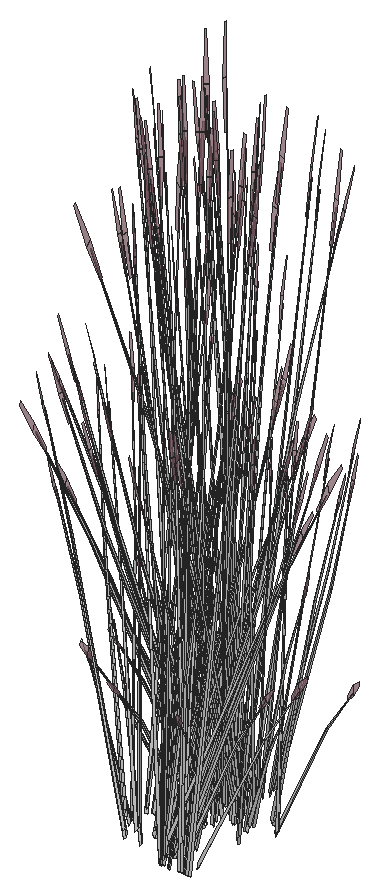
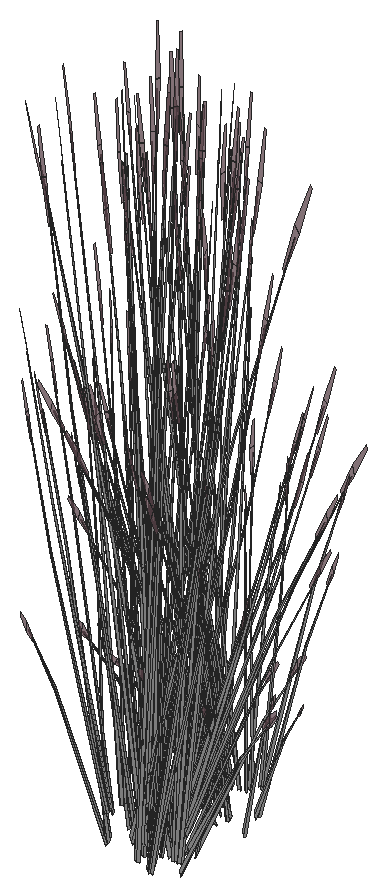
# SketchUp Ruby script. Lengths in inches.
U = 1.inch
M = Sketchup.active_model
def pt(a) = Geom::Point3d.new(a.map { |v| v * U })
def face(e, loops, mat)
  f = e.add_face(loops[0].map { |a| pt(a) })
  loops[1..].each { |l| e.add_face(l.map { |a| pt(a) }).erase! }
  f.material = f.back_material = mat if mat
  f
end
# faces: each face lists its corners as indices into pts; further lists are holes
def faces(e, pts, list, mat = nil) = list.each { |f| face(e, (f[0].is_a?(Array) ? f : [f]).map { |l| l.map { |i| pts[i] } }, mat) }
# xy, xz, yz: faces in a plane at the given z, y or x. An outline is a flat list of corners, or four numbers for a rectangle; further outlines are holes
def ring(l) = l.size == 4 ? [[l[0], l[1]], [l[2], l[1]], [l[2], l[3]], [l[0], l[3]]] : l.each_slice(2).to_a
def flat(e, list, mat, &to3) = list.each { |f| face(e, (f[0].is_a?(Array) ? f : [f]).map { |l| ring(l).map { |u, v| to3.(u, v) } }, mat) }
def xy(e, z, list, mat = nil) = flat(e, list, mat) { |x, y| [x, y, z] }
def xz(e, y, list, mat = nil) = flat(e, list, mat) { |x, z| [x, y, z] }
def yz(e, x, list, mat = nil) = flat(e, list, mat) { |y, z| [x, y, z] }
def lines(e, pts, list) = list.each { |a, b| e.add_line(pt(pts[a]), pt(pts[b])) }
# prism: a flat outline (further loops are holes) pulled along v
def prism(e, loops, v, mat = nil)
  f = face(e, loops, mat); d = Geom::Vector3d.new(v.map { |x| x * U })
  f.pushpull(f.normal.samedirection?(d) ? d.length : -d.length)
end
def box(e, o, s, mat = nil) = prism(e, [[o, [o[0] + s[0], o[1], o[2]], [o[0] + s[0], o[1] + s[1], o[2]], [o[0], o[1] + s[1], o[2]]]], [0, 0, s[2]], mat)
def at(x, y, z, deg = 0) = Geom::Transformation.translation(pt([x, y, z])) * Geom::Transformation.rotation(ORIGIN, Z_AXIS, deg.degrees)
def axes(o, x, y, z) = Geom::Transformation.new([*x, 0, *y, 0, *z, 0, *pt(o).to_a, 1])
def part(name) = M.definitions.add(name)
# library, detail: a bought-in or finely detailed component or shape, given as its bounding box
def library(name, o, s) = part(name).tap { |d| box(d.entities, o, s) }
def detail(e, o, s) = box(e.add_group.entities, o, s)
def put(e, d, t, mat = nil) = e.add_instance(d, t).tap { |i| i.material = mat if mat }
def group(e, t, mat = nil) = e.add_group.tap { |g| g.transformation = t; g.material = mat if mat }.entities
root = M.entities
M.materials.add("LightPink_Translucent").color = [144, 107, 117]
M.materials["LightPink_Translucent"].alpha = 0.75
M.materials.add("[_0053_Ivory_]").color = [200, 200, 200]
c1 = part("blade")
p = [[2.15,0.21,22],[0,0.17,0],[0.09,0.45,0],[2.18,0.31,22],[2.29,0.31,22],[0.38,0.45,0],
  [2.48,0.24,33],[2.49,0.24,33],[2.48,0.22,33]]
faces(c1.entities,p,[[0,1,2,3],[4,5,2,3],[6,3,4,7],[8,0,3,6]])
c2 = part("seeds")
p = [[0.3,-0.1,1.38],[-0.01,-0.03,1.59],[-0.01,-0.03,0.03],[0.14,-0.07,-0.07],[0.29,-0.03,3],[0.15,0.01,3.11]]
faces(c2.entities,p,[[0,1,2,3],[1,0,4,5]],"LightPink_Translucent")
c3 = part("blade with seeds")
put(c3.entities,c1,at(0,0,0))
put(c3.entities,c2,axes([2.4,0.25,30.99],[1.5799,-0.05474,1.17369],[-0.12525,1.92788,0.29478],[-0.07173,-0.02425,1.56792]))
put(root,c3,axes([629.1875,284.57,255.53],[0.21074,-0.13302,1.71376],[0.17741,0.61464,0.13857],[-0.33083,0.13891,0.73262]),"[_0053_Ivory_]")
put(root,c3,axes([633.4,292.35,256.63],[0.0158,-0.58168,-0.71045],[0.66548,0.03907,0.08574],[0.07023,-0.24643,1.00501]),"[_0053_Ivory_]")
put(root,c3,axes([632.25,291.42,256.18],[0.1831,-0.48359,-0.35414],[0.53419,0.14105,0.4572],[-0.04898,-0.1947,0.87481]),"[_0053_Ivory_]")
put(root,c3,axes([632.65,292.06,255.53],[-0.11309,0.21615,1.71376],[-0.47441,-0.44731,0.13857],[0.21402,-0.27879,0.73262]),"[_0053_Ivory_]")
put(root,c3,axes([633.82,285.9375,256.63],[0.60713,0.01514,-0.71045],[-0.04078,0.63759,0.08574],[0.25721,0.06729,1.00501]),"[_0053_Ivory_]")
put(root,c3,axes([633.13,286.45,254.13],[0.56842,-0.31443,0.49651],[0.33976,0.56381,0],[-0.12946,0.07161,1.57504]),"[_0053_Ivory_]")
put(root,c3,axes([631.98,291.75,256.33],[-0.59704,-0.15764,-0.51099],[0.20464,-0.54049,-0.3958],[-0.05475,-0.21761,0.97773]),"[_0053_Ivory_]")
put(root,c3,axes([632.35,290.4,254.42],[0.07791,0.3667,1.1486],[-0.43222,-0.2031,0.84392],[0.04651,-0.18776,0.25299]),"[_0053_Ivory_]")
put(root,c3,axes([632.32,285.95,253.94],[0.26406,0.72244,-0.06012],[-0.7545,0.25315,0],[0.00922,0.02523,1.72173]),"[_0053_Ivory_]")
put(root,c3,axes([632.62,286.73,253.68],[-0.56663,-0.1556,-0.30978],[0.14267,-0.54795,0.30978],[-0.11423,0.06319,1.38974]),"[_0053_Ivory_]")
put(root,c3,axes([633.27,292.16,256.33],[-0.43478,-0.42253,-0.51099],[0.45929,-0.37004,-0.3958],[0.06615,-0.21468,0.97773]),"[_0053_Ivory_]")
put(root,c3,axes([628.53,285.62,254.24],[0.21107,0.05162,1.43002],[0.13604,0.52729,-0.30754],[-0.28671,0.0987,0.61141]),"[_0053_Ivory_]")
put(root,c3,axes([634.81,284.64,254.03],[0.75945,0,0],[0,0.70283,-0.51607],[0,0.16007,1.63711]),"[_0053_Ivory_]")
put(root,c3,axes([634.51,285,253.85],[-0.75908,-0.00503,-0.04976],[0,-0.70283,0.49943],[-0.02386,0.16,1.58352]),"[_0053_Ivory_]")
put(root,c3,axes([632.86,284.39,254.32],[0.68399,0.30005,-0.29095],[-0.32934,0.63331,-0.50002],[0.0215,0.15549,1.59708]),"[_0053_Ivory_]")
put(root,c3,axes([628.09,286.73,254.42],[0.25312,-0.28501,1.1486],[0.09988,0.45119,0.84392],[-0.18292,0.08079,0.25299]),"[_0053_Ivory_]")
put(root,c3,axes([634.18,286.2,256.18],[0.34557,0.39372,-0.35414],[-0.39459,0.37271,0.4572],[0.20048,0.05671,0.87481]),"[_0053_Ivory_]")
put(root,c3,axes([634.35,285.11,253.68],[-0.42396,0.39235,-0.30978],[-0.42396,-0.39235,0.30978],[0,0.12637,1.38974]),"[_0053_Ivory_]")
put(root,c3,axes([632.52,285.14,254.32],[0.07077,0.71755,-0.29095],[-0.73712,0.04339,-0.50002],[-0.1298,0.09558,1.59708]),"[_0053_Ivory_]")
put(root,c3,axes([632.79,284.86,253.86],[-0.29468,0.56664,-0.44739],[-0.61229,-0.27271,0.21531],[0,0.13062,1.43643]),"[_0053_Ivory_]")
put(root,c3,axes([629.04,285.49,256.18],[-0.52868,0.08987,-0.35414],[-0.1396,-0.51376,0.4572],[-0.1515,0.13799,0.87481]),"[_0053_Ivory_]")
put(root,c3,axes([633.68,292,256.18],[0.41095,-0.33109,-0.35414],[0.38901,0.37805,0.4572],[0.05919,-0.19208,0.87481]),"[_0053_Ivory_]")
put(root,c3,axes([630.125,290.84,254.42],[0.31682,0.21887,1.1486],[-0.4614,0.13157,0.84392],[-0.09872,-0.16821,0.25299]),"[_0053_Ivory_]")
put(root,c3,axes([630.89,292,256.63],[-0.51789,-0.30395,-0.71045],[0.36805,-0.53263,0.08574],[-0.18764,-0.18149,1.00501]),"[_0053_Ivory_]")
put(root,c3,axes([630.71,291.6,256.18],[-0.0938,-0.50652,-0.35414],[0.53623,-0.13375,0.4572],[-0.14403,-0.14515,0.87481]),"[_0053_Ivory_]")
put(root,c3,axes([632.08,285.69,253.71],[-0.40909,0.47266,-0.62353],[-0.50819,-0.4286,-0.16365],[-0.16393,0.11791,1.37633]),"[_0053_Ivory_]")
put(root,c3,axes([632.81,286.49,253.98],[0.76036,0.2044,0.30756],[-0.19023,0.7306,-0.36492],[-0.12585,0.09144,1.64885]),"[_0053_Ivory_]")
put(root,c3,axes([632.75,286.98,253.67],[-0.56842,0.31443,-0.49651],[-0.33976,-0.56381,0],[-0.12946,0.07161,1.57504]),"[_0053_Ivory_]")
put(root,c3,axes([634.64,285.12,253.67],[0,0.62885,-0.49651],[-0.67951,0,0],[0,0.14322,1.57504]),"[_0053_Ivory_]")
put(root,c3,axes([632.94,285.19,255.53],[-0.2256,-0.10835,1.71376],[0.46687,-0.45453,0.13857],[0.29098,0.20505,0.73262]),"[_0053_Ivory_]")
put(root,c3,axes([629.875,291.5,253.15],[-0.05883,0.08284,1.76342],[-0.59454,0.17861,-0.26939],[-0.14363,-0.16248,0.30037]),"[_0053_Ivory_]")
put(root,c3,axes([630.86,293.77,253.75],[-0.24943,-0.64486,-0.69835],[0.71849,-0.23224,-0.18329],[-0.02757,-0.21836,1.54149]),"[_0053_Ivory_]")
put(root,c3,axes([629.56,292.33,255.53],[0.2256,0.10835,1.71376],[-0.46687,0.45453,0.13857],[-0.29098,-0.20505,0.73262]),"[_0053_Ivory_]")
put(root,c3,axes([634.19,291.8,253.15],[-0.0909,-0.04954,1.76342],[-0.2335,-0.55347,-0.26939],[0.15752,-0.1502,0.30037]),"[_0053_Ivory_]")
put(root,c3,axes([633.78,286.42,254.42],[-0.34197,-0.18082,1.1486],[0.44156,-0.18372,0.84392],[0.1191,0.15563,0.25299]),"[_0053_Ivory_]")
put(root,c3,axes([629.96,284.99,255.53],[0.1517,-0.19322,1.71376],[0.38303,0.52154,0.13857],[-0.26271,0.23751,0.73262]),"[_0053_Ivory_]")
put(root,c3,axes([630.65,292.01,256.33],[-0.59932,0.14948,-0.51099],[-0.10484,-0.56611,-0.3958],[-0.16097,-0.16223,0.97773]),"[_0053_Ivory_]")
put(root,c3,axes([629.48,285.55,256.33],[0.15602,0.5742,-0.51099],[-0.59087,0.10045,-0.3958],[-0.16933,0.15423,0.97773]),"[_0053_Ivory_]")
put(root,c3,axes([633.27,286.88,254.03],[0.37973,0.63014,0],[-0.6353,0.35142,-0.51607],[-0.14469,0.08004,1.63711]),"[_0053_Ivory_]")
put(root,c3,axes([633.87,287.1,253.15],[0.04425,-0.09079,1.76342],[0.55709,-0.26738,-0.26939],[0.16889,0.13839,0.30037]),"[_0053_Ivory_]")
put(root,c3,axes([632.94,284.39,254.5],[-0.01659,-0.59209,1.41272],[0.75089,0.15348,0.59816],[-0.1776,0.32398,1.3335]),"[_0053_Ivory_]")
put(root,c3,axes([633.14,285.03,253.75],[0.2227,0.57576,-0.69212],[-0.64151,0.20736,-0.18165],[0.02462,0.19497,1.52773]),"[_0053_Ivory_]")
put(root,c3,axes([634.1875,293.37,256.63],[0.31725,-0.49618,-0.71045],[0.55593,0.35263,0.08574],[0.18942,-0.17977,1.00501]),"[_0053_Ivory_]")
put(root,c3,axes([628.76,287.02,253.15],[0.08147,0.06283,1.76342],[0.13814,0.58211,-0.26939],[-0.18056,0.12413,0.30037]),"[_0053_Ivory_]")
put(root,c3,axes([630.76,291.92,254.03],[-0.37973,-0.63014,0],[0.6353,-0.35142,-0.51607],[0.14469,-0.08004,1.63711]),"[_0053_Ivory_]")
put(root,c3,axes([634.17,293.13,256.33],[-0.15602,-0.5742,-0.51099],[0.59087,-0.10045,-0.3958],[0.16933,-0.15423,0.97773]),"[_0053_Ivory_]")
put(root,c3,axes([633,286.67,256.33],[0.59932,-0.14948,-0.51099],[0.10484,0.56611,-0.3958],[0.16097,0.16223,0.97773]),"[_0053_Ivory_]")
put(root,c3,axes([631.59,291.16,253.78],[-0.4197,0.36076,-0.03893],[-0.38456,-0.39511,-0.17649],[-0.02707,-0.11196,0.58215]),"[_0053_Ivory_]")
put(root,c3,axes([633.83,287.25,254.32],[-0.38947,-0.01972,1.0506],[0.25721,-0.41888,0.58006],[0.15386,0.14882,0.8241]),"[_0053_Ivory_]")
put(root,c3,axes([632.13,295.4375,254.98],[0.52485,0.25358,1.51261],[-0.51417,0.54629,0.59816],[-0.23031,-0.32378,1.26806]),"[_0053_Ivory_]")
put(root,c3,axes([629.39,293.68,253.67],[0,-0.62885,-0.49651],[0.67951,0,0],[0,-0.14322,1.57504]),"[_0053_Ivory_]")
put(root,c3,axes([631.27,291.82,253.67],[0.56842,-0.31443,-0.49651],[0.33976,0.56381,0],[0.12946,-0.07161,1.57504]),"[_0053_Ivory_]")
put(root,c3,axes([634.65,292.91,254.24],[-0.21697,-0.01863,1.43002],[-0.22228,-0.49966,-0.30754],[0.26655,-0.14135,0.61141]),"[_0053_Ivory_]")
put(root,c3,axes([629.84,285.46,255.53],[0.11309,-0.21615,1.71376],[0.47441,0.44731,0.13857],[-0.21402,0.27879,0.73262]),"[_0053_Ivory_]")
put(root,c3,axes([631.95,293.11,253.71],[0.40909,-0.47266,-0.62353],[0.50819,0.4286,-0.16365],[0.16393,-0.11791,1.37633]),"[_0053_Ivory_]")
put(root,c3,axes([632.56,286.23,254.24],[0.01072,-0.20846,1.43002],[0.51218,-0.23285,-0.30754],[0.15811,0.2495,0.61141]),"[_0053_Ivory_]")
put(root,c3,axes([634.9,291.99,254.42],[-0.2023,0.32011,1.1486],[-0.17388,-0.43009,0.84392],[0.16708,-0.10777,0.25299]),"[_0053_Ivory_]")
put(root,c3,axes([629.97,286.68,256.18],[-0.41095,0.33109,-0.35414],[-0.38901,-0.37805,0.4572],[-0.05919,0.19208,0.87481]),"[_0053_Ivory_]")
put(root,c3,axes([634.61,293.19,256.18],[0.52868,-0.08987,-0.35414],[0.1396,0.51376,0.4572],[0.1515,-0.13799,0.87481]),"[_0053_Ivory_]")
put(root,c3,axes([630.24,287.97,254.42],[-0.01572,-0.37392,1.1486],[0.39276,0.26669,0.84392],[-0.07724,0.17822,0.25299]),"[_0053_Ivory_]")
put(root,c3,axes([631.24,293.94,253.86],[0.29468,-0.56664,-0.44739],[0.61229,0.27271,0.21531],[0,-0.13062,1.43643]),"[_0053_Ivory_]")
put(root,c3,axes([629.47,292.49,256.18],[-0.34557,-0.39372,-0.35414],[0.39459,-0.37271,0.4572],[-0.20048,-0.05671,0.87481]),"[_0053_Ivory_]")
put(root,c3,axes([631.5,293.66,254.32],[-0.07077,-0.71755,-0.29095],[0.73712,-0.04339,-0.50002],[0.1298,-0.09558,1.59708]),"[_0053_Ivory_]")
put(root,c3,axes([631.27,287.08,253.15],[0.09829,-0.03422,1.76342],[0.59126,0.18834,-0.26939],[0.01729,0.21228,0.30037]),"[_0053_Ivory_]")
put(root,c3,axes([629.68,293.7,253.68],[0.42396,-0.39235,-0.30978],[0.42396,0.39235,0.30978],[0,-0.12637,1.38974]),"[_0053_Ivory_]")
put(root,c3,axes([629.51,291.82,253.78],[-0.1752,0.51349,-0.03893],[-0.53924,-0.15795,-0.17649],[-0.08187,-0.08399,0.58215]),"[_0053_Ivory_]")
put(root,c3,axes([631.16,294.41,254.32],[-0.68399,-0.30005,-0.29095],[0.32934,-0.63331,-0.50002],[-0.0215,-0.15549,1.59708]),"[_0053_Ivory_]")
put(root,c3,axes([630.38,286.53,256.66],[0.43478,0.42253,-0.5672],[-0.45929,0.37004,-0.43934],[-0.06615,0.21468,1.08528]),"[_0053_Ivory_]")
put(root,c3,axes([629.22,294.16,254.03],[-0.75945,0,0],[0,-0.70283,-0.51607],[0,-0.16007,1.63711]),"[_0053_Ivory_]")
put(root,c3,axes([629.35,292.91,254.24],[0.11858,0.17508,1.43002],[-0.27325,0.4759,-0.30754],[-0.28057,-0.11375,0.61141]),"[_0053_Ivory_]")
put(root,c3,axes([629.91,287.16,254.48],[0.55175,-0.11136,0.06507],[0.12684,0.44864,-0.86304],[-0.03498,0.22711,0.7736]),"[_0053_Ivory_]")
put(root,c3,axes([631.67,286.94,256.33],[0.59704,0.15764,-0.51099],[-0.20464,0.54049,-0.3958],[0.05475,0.21761,0.97773]),"[_0053_Ivory_]")
put(root,c3,axes([632.01,285.82,255.53],[-0.13883,-0.2019,1.71376],[0.64153,-0.16998,0.13857],[0.14499,0.31697,0.73262]),"[_0053_Ivory_]")
put(root,c3,axes([631.41,292.07,253.68],[0.56663,0.1556,-0.30978],[-0.14267,0.54795,0.30978],[0.11423,-0.06319,1.38974]),"[_0053_Ivory_]")
put(root,c3,axes([629.83,292.75,256.63],[-0.60713,-0.01514,-0.71045],[0.04078,-0.63759,0.08574],[-0.25721,-0.06729,1.00501]),"[_0053_Ivory_]")
put(root,c3,axes([631.4,287.27,256.18],[-0.1831,0.48359,-0.35414],[-0.53419,-0.14105,0.4572],[0.04898,0.1947,0.87481]),"[_0053_Ivory_]")
put(root,c3,axes([630.25,286.33,256.99],[-0.0158,0.58168,-0.7886],[-0.66548,-0.03907,0.09517],[-0.07023,0.24643,1.11556]),"[_0053_Ivory_]")
put(root,c3,axes([630.88,285.92,255.53],[-0.01487,-0.24136,1.71376],[0.64429,0.16012,0.13857],[-0.03985,0.34396,0.73262]),"[_0053_Ivory_]")
put(root,c3,axes([629.8,293.98,253.98],[-0.56493,0.5287,0.30756],[-0.56528,-0.52313,-0.36492],[-0.01973,-0.15014,1.64885]),"[_0053_Ivory_]")
put(root,c3,axes([631.46,286.83,256.63],[0.28988,0.51132,-0.71045],[-0.59671,0.28496,0.08574],[0.06778,0.24706,1.00501]),"[_0053_Ivory_]")
put(root,c3,axes([631.6,294.22,254.09],[0.68433,0.30479,0.24065],[-0.32934,0.63331,0.50002],[0,-0.14599,1.60543]),"[_0053_Ivory_]")
put(root,c3,axes([631.33,295.08,254.09],[0.16098,-0.74515,-0.23429],[0.76326,0.12989,0.51271],[-0.13337,-0.1029,1.5644]),"[_0053_Ivory_]")
put(root,c3,axes([629.63,292.88,256.33],[-0.44101,0.41656,-0.51099],[-0.38623,-0.44004,-0.3958],[-0.22407,-0.06338,0.97773]),"[_0053_Ivory_]")
put(root,c3,axes([629.78,287.64,254.24],[0.19166,-0.0992,1.43002],[0.4732,0.29912,-0.30754],[-0.14084,0.25882,0.61141]),"[_0053_Ivory_]")
put(root,c3,axes([628.64,293.43,254.42],[0.38775,-0.045,1.1486],[-0.24596,0.39648,0.84392],[-0.19161,-0.05948,0.25299]),"[_0053_Ivory_]")
put(root,c3,axes([631.38,293.8,254.37],[-0.65953,0.03882,0.44739],[-0.05964,-0.64439,-0.21531],[0.11807,-0.06531,1.43643]),"[_0053_Ivory_]")
put(root,c3,axes([629.68,294.27,254.13],[0,0.62885,0.49651],[-0.67951,0,0],[0,-0.14322,1.57504]),"[_0053_Ivory_]")
put(root,c3,axes([634.45,294.41,256.33],[0.16454,-0.57202,-0.51099],[0.56413,0.19607,-0.3958],[0.22713,-0.05245,0.97773]),"[_0053_Ivory_]")
put(root,c3,axes([633.55,292.08,254.03],[0.37973,-0.63014,0],[0.6353,0.35142,-0.51607],[0.14469,0.08004,1.63711]),"[_0053_Ivory_]")
put(root,c3,axes([629.08,293.32,255.53],[0.25192,-0.01424,1.71376],[-0.16712,0.61729,0.13857],[-0.35901,-0.03818,0.73262]),"[_0053_Ivory_]")
put(root,c3,axes([631.28,294.78,253.86],[-0.36485,-0.52782,-0.44739],[0.55265,-0.37168,0.21531],[-0.11807,-0.06531,1.43643]),"[_0053_Ivory_]")
put(root,c3,axes([631.36,294.03,254.01],[0.26406,0.70318,0.45755],[-0.7545,0.24452,0.17955],[0.00922,-0.12921,1.58856]),"[_0053_Ivory_]")
put(root,c3,axes([635.05,294.57,253.64],[-0.39118,0.07547,1.41583],[-0.06226,-0.6007,0.08104],[0.27398,-0.09092,0.80566]),"[_0053_Ivory_]")
put(root,c3,axes([635.76,294.04,253.91],[-0.37654,-0.40212,-0.06488],[0.4124,-0.36845,-0.29416],[0.11685,-0.02594,0.97024]),"[_0053_Ivory_]")
put(root,c3,axes([631.22,294.58,254.37],[-0.29468,0.56664,0.44739],[-0.61229,-0.27271,-0.21531],[0,-0.13062,1.43643]),"[_0053_Ivory_]")
put(root,c3,axes([630.03,287.15,255.02],[0.01334,-0.32463,1.54345],[0.60018,0.17147,0.21329],[-0.052,0.34598,0.72882]),"[_0053_Ivory_]")
put(root,c3,axes([632.31,294.09,253.86],[0,-0.72763,0],[0.75945,0,0],[0,0,1.79456]),"[_0053_Ivory_]")
put(root,c3,axes([633.23,292.41,254.13],[-0.56842,-0.31443,0.49651],[0.33976,-0.56381,0],[0.12946,0.07161,1.57504]),"[_0053_Ivory_]")
put(root,c3,axes([634.34,294.62,256.63],[0.53369,-0.27773,-0.71045],[0.29743,0.5717,0.08574],[0.25786,-0.06494,1.00501]),"[_0053_Ivory_]")
put(root,c3,axes([630.95,294.98,253.71],[-0.63179,-0.1031,-0.62353],[0.13332,-0.63596,-0.16365],[-0.18854,-0.07706,1.37633]),"[_0053_Ivory_]")
put(root,c3,axes([631.95,293.63,254.01],[-0.50358,0.57069,0.45755],[-0.59827,-0.50377,0.17955],[0.1214,-0.05695,1.58856]),"[_0053_Ivory_]")
put(root,c3,axes([632.5,294.65,253.95],[-0.56493,-0.54126,-0.06131],[0.56528,-0.54159,0],[-0.01973,-0.0189,1.75571]),"[_0053_Ivory_]")
put(root,c3,axes([631.07,292.69,254.13],[-0.17545,0.62497,0.17642],[-0.64204,-0.17686,0.35086],[0.11091,-0.00304,1.60407]),"[_0053_Ivory_]")
put(root,c3,axes([630.81,293.2,253.25],[-0.59782,0.25177,1.28929],[-0.19028,-0.72239,0.50096],[0.36709,0.01202,1.46642]),"[_0053_Ivory_]")
put(root,c3,axes([632.41,293.39,254.27],[0.11717,-0.56122,0.1448],[0.57245,0.09742,-0.41347],[0.10418,0.05763,1.26744]),"[_0053_Ivory_]")
put(root,c3,axes([631.42,294.72,254.01],[0.76764,0.13249,0.45755],[-0.15622,0.74829,0.17955],[-0.11218,-0.07226,1.58856]),"[_0053_Ivory_]")
put(root,c3,axes([635.48,294.18,253.15],[-0.03174,-0.09547,1.76342],[0.22015,-0.55846,-0.26939],[0.22208,-0.00803,0.30037]),"[_0053_Ivory_]")
put(root,c3,axes([628.92,294.08,253.15],[0.0154,0.09911,1.76342],[-0.31051,0.51756,-0.26939],[-0.22056,-0.02609,0.30037]),"[_0053_Ivory_]")
put(root,c3,axes([632.17,293.53,254.37],[-0.36485,-0.52782,0.44739],[0.55265,-0.37168,-0.21531],[0.11807,0.06531,1.43643]),"[_0053_Ivory_]")
put(root,c3,axes([630.28,295.95,253.68],[-0.14267,-0.54795,-0.30978],[0.56663,-0.1556,0.30978],[-0.11423,-0.06319,1.38974]),"[_0053_Ivory_]")
put(root,c3,axes([631.01,295.91,254.13],[0.65264,-0.16691,0.17642],[0.16115,0.62115,0.35086],[-0.05821,-0.0905,1.60407]),"[_0053_Ivory_]")
put(root,c3,axes([632.35,293.57,254.32],[0.61322,-0.4175,-0.29095],[0.40778,0.58992,-0.50002],[0.1513,0.05991,1.59708]),"[_0053_Ivory_]")
put(root,c3,axes([634.79,294.67,256.18],[0.50475,0.17543,-0.35414],[-0.14722,0.5118,0.4572],[0.20322,-0.04693,0.87481]),"[_0053_Ivory_]")
put(root,c3,axes([630.125,296.18,253.67],[-0.56842,-0.31443,-0.49651],[0.33976,-0.56381,0],[-0.12946,-0.07161,1.57504]),"[_0053_Ivory_]")
put(root,c3,axes([633.9,292.46,253.67],[0.56842,0.31443,-0.49651],[-0.33976,0.56381,0],[0.12946,0.07161,1.57504]),"[_0053_Ivory_]")
